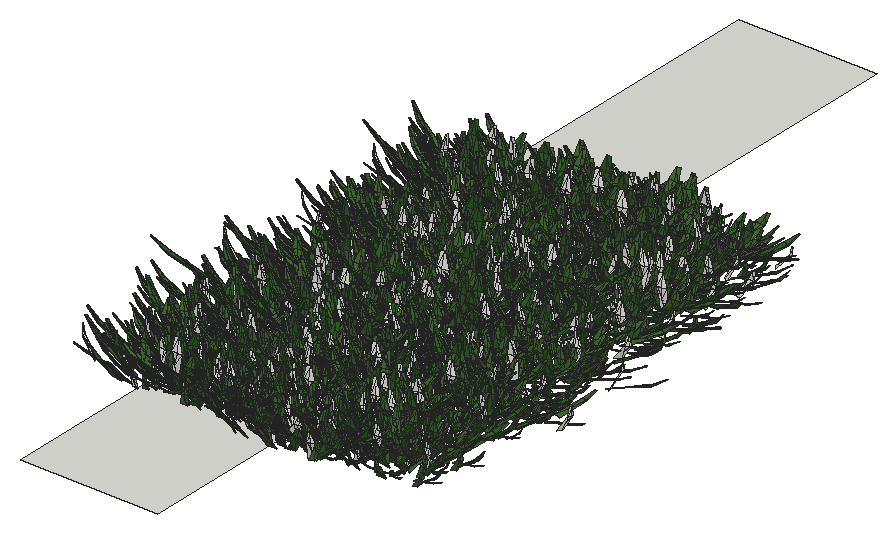
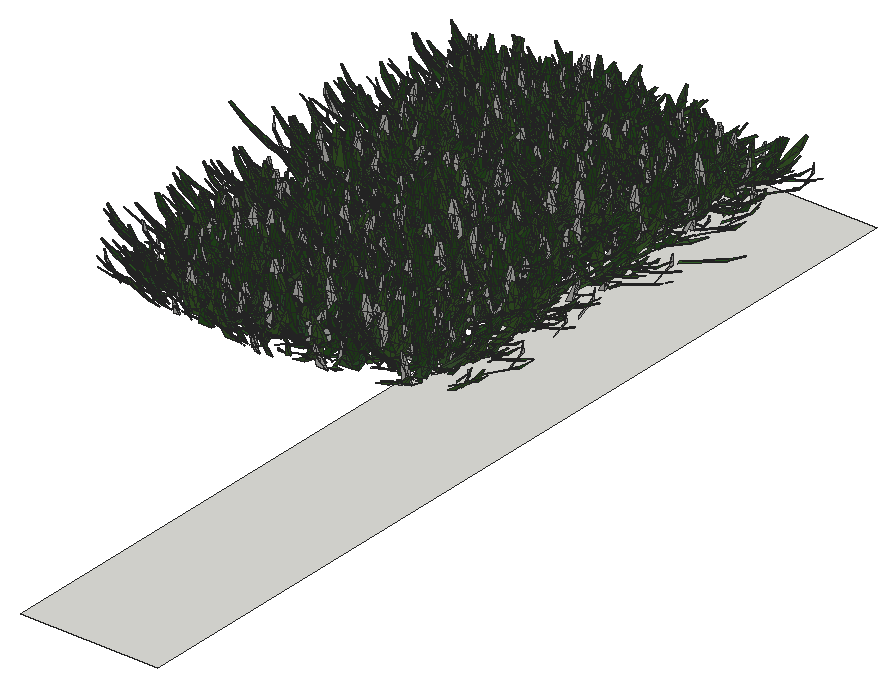
# SketchUp Ruby script. Lengths in inches.
U = 1.inch
M = Sketchup.active_model
def pt(a) = Geom::Point3d.new(a.map { |v| v * U })
def face(e, loops, mat)
  f = e.add_face(loops[0].map { |a| pt(a) })
  loops[1..].each { |l| e.add_face(l.map { |a| pt(a) }).erase! }
  f.material = f.back_material = mat if mat
  f
end
# faces: each face lists its corners as indices into pts; further lists are holes
def faces(e, pts, list, mat = nil) = list.each { |f| face(e, (f[0].is_a?(Array) ? f : [f]).map { |l| l.map { |i| pts[i] } }, mat) }
# xy, xz, yz: faces in a plane at the given z, y or x. An outline is a flat list of corners, or four numbers for a rectangle; further outlines are holes
def ring(l) = l.size == 4 ? [[l[0], l[1]], [l[2], l[1]], [l[2], l[3]], [l[0], l[3]]] : l.each_slice(2).to_a
def flat(e, list, mat, &to3) = list.each { |f| face(e, (f[0].is_a?(Array) ? f : [f]).map { |l| ring(l).map { |u, v| to3.(u, v) } }, mat) }
def xy(e, z, list, mat = nil) = flat(e, list, mat) { |x, y| [x, y, z] }
def xz(e, y, list, mat = nil) = flat(e, list, mat) { |x, z| [x, y, z] }
def yz(e, x, list, mat = nil) = flat(e, list, mat) { |y, z| [x, y, z] }
def lines(e, pts, list) = list.each { |a, b| e.add_line(pt(pts[a]), pt(pts[b])) }
# prism: a flat outline (further loops are holes) pulled along v
def prism(e, loops, v, mat = nil)
  f = face(e, loops, mat); d = Geom::Vector3d.new(v.map { |x| x * U })
  f.pushpull(f.normal.samedirection?(d) ? d.length : -d.length)
end
def box(e, o, s, mat = nil) = prism(e, [[o, [o[0] + s[0], o[1], o[2]], [o[0] + s[0], o[1] + s[1], o[2]], [o[0], o[1] + s[1], o[2]]]], [0, 0, s[2]], mat)
def at(x, y, z, deg = 0) = Geom::Transformation.translation(pt([x, y, z])) * Geom::Transformation.rotation(ORIGIN, Z_AXIS, deg.degrees)
def axes(o, x, y, z) = Geom::Transformation.new([*x, 0, *y, 0, *z, 0, *pt(o).to_a, 1])
def part(name) = M.definitions.add(name)
# library, detail: a bought-in or finely detailed component or shape, given as its bounding box
def library(name, o, s) = part(name).tap { |d| box(d.entities, o, s) }
def detail(e, o, s) = box(e.add_group.entities, o, s)
def put(e, d, t, mat = nil) = e.add_instance(d, t).tap { |i| i.material = mat if mat }
def group(e, t, mat = nil) = e.add_group.tap { |g| g.transformation = t; g.material = mat if mat }.entities
root = M.entities
M.materials.add("Material82").color = [68, 110, 58]
M.materials.add("Material83").color = [48, 90, 38]
M.materials.add("Material84").color = [68, 110, 48]
M.materials.add("Material85").color = [48, 90, 48]
M.materials.add("Material86").color = [58, 110, 58]
M.materials.add("Material87").color = [58, 90, 38]
M.materials.add("Material88").color = [68, 100, 58]
M.materials.add("Material89").color = [48, 100, 38]
c1 = part("grass00")
p = [[-0.6875,0.15,0],[-0.56,0.08,5.52],[-0.04,0.03,2.76],[0.48,-0.02,0],[0.35,-0.02,5.52],[-0.1,-0.14,5.52],
  [-0.12,0.65,8.37],[-0.42,0.65,8.37]]
faces(c1.entities,p,[[0,1,2,3],[3,2,4],[1,5,2],[5,4,2],[1,6,5],[4,5,6],[7,6,1]])
c2 = part("Group16\#1")
put(c2.entities,c1,axes([1.44,-0.61,-0.01],[0.05352,0.12609,0],[-0.10704,0.04543,0.07239],[0.06664,-0.02828,0.11628]),"Material85")
put(c2.entities,c1,axes([0.76,-0.15,-0.01],[0.04676,0.24062,0],[-0.23162,0.04501,0.06642],[0.0652,-0.01267,0.23595]),"Material82")
put(c2.entities,c1,axes([0.79,0.01,-0.01],[-0.00606,0.34651,0],[-0.34381,-0.00602,0.0432],[0.04319,0.00076,0.34386]))
put(c2.entities,c1,axes([1,0.23,-0.01],[-0.07192,0.31144,0],[-0.28722,-0.06632,0.1236],[0.12043,0.02781,0.29478]),"Material84")
put(c2.entities,c1,axes([1.66,0.77,-0.01],[-0.13828,0.29651,0],[-0.21551,-0.1005,0.22471],[0.20365,0.09498,0.23779]),"Material89")
put(c2.entities,c1,axes([0.6875,0.52,-0.01],[-0.18126,0.24051,0],[-0.22746,-0.17142,0.09788],[0.07817,0.05891,0.28481]),"Material84")
put(c2.entities,c1,axes([0.68,0.78,-0.01],[-0.215,0.18688,0],[-0.12385,-0.14248,0.21334],[0.13995,0.16101,0.18878]),"Material82")
put(c2.entities,c1,axes([0.56,1,-0.01],[-0.13756,0.07624,0],[-0.06159,-0.11112,0.0927],[0.04494,0.08108,0.12705]),"Material84")
put(c2.entities,c1,axes([0.2,0.64,-0.01],[-0.23729,0.07254,0],[-0.05711,-0.18681,0.153],[0.04473,0.14632,0.19535]),"Material89")
put(c2.entities,c1,axes([0.0625,0.72,-0.01],[-0.28874,0.02525,0],[-0.02179,-0.24916,0.14647],[0.01276,0.14591,0.25012]),"Material82")
put(c2.entities,c1,axes([-0.08,0.62,-0.01],[-0.34089,-0.04187,0],[0.03255,-0.26504,0.216],[-0.02633,0.21439,0.26703]),"Material89")
put(c2.entities,c1,axes([-0.34,0.98,-0.01],[-0.14314,-0.0493,0],[0.04397,-0.12769,0.06843],[-0.02228,0.0647,0.13505]),"Material89")
put(c2.entities,c1,axes([-0.87,1.45,-0.01],[-0.23488,-0.14114,0],[0.13761,-0.22901,0.06087],[-0.03135,0.05217,0.26717]))
put(c2.entities,c1,axes([-0.72,0.77,-0.01],[-0.14208,-0.13251,0],[0.07209,-0.0773,0.16301],[-0.11118,0.11922,0.1057]),"Material89")
put(c2.entities,c1,axes([-0.62,0.43,-0.01],[-0.14845,-0.21203,0],[0.18654,-0.13061,0.12304],[-0.10079,0.07057,0.22772]),"Material82")
put(c2.entities,c1,axes([-0.68,0.29,-0.01],[-0.13639,-0.32136,0],[0.31723,-0.13464,0.05579],[-0.05136,0.0218,0.34462]),"Material83")
put(c2.entities,c1,axes([-0.64,0.125,-0.01],[-0.0458,-0.23569,0],[0.22124,-0.043,0.08276],[-0.08124,0.01579,0.22538]),"Material86")
put(c2.entities,c1,axes([-1.6,-0.03,-0.01],[0.00576,-0.32897,0],[0.27526,0.00482,0.18018],[-0.18015,-0.00315,0.2753]),"Material84")
put(c2.entities,c1,axes([-1.36,-0.31,-0.01],[0.05718,-0.24765,0],[0.18172,0.04196,0.17267],[-0.16825,-0.03885,0.1865]),"Material89")
put(c2.entities,c1,axes([-1.54,-0.72,-0.01],[0.06537,-0.14017,0],[0.13555,0.06321,0.03939],[-0.0357,-0.01665,0.14956]))
put(c2.entities,c1,axes([-1.19,-0.9,-0.01],[0.09597,-0.12735,0],[0.11214,0.08451,0.07557],[-0.06035,-0.04548,0.14042]),"Material88")
put(c2.entities,c1,axes([-0.47,-0.54,-0.01],[0.11588,-0.10072,0],[0.0618,0.0711,0.12124],[-0.07953,-0.0915,0.0942]))
put(c2.entities,c1,axes([-0.47,-0.84,-0.01],[0.11927,-0.0661,0],[0.06603,0.11913,0.00646],[-0.00313,-0.00565,0.13621]),"Material84")
put(c2.entities,c1,axes([-0.38,-1.24,-0.01],[0.28037,-0.08571,0],[0.0618,0.20215,0.20315],[-0.05939,-0.19428,0.21139]),"Material88")
put(c2.entities,c1,axes([-0.06,-0.66,-0.01],[0.22719,-0.01987,0],[0.01247,0.14255,0.17758],[-0.01547,-0.17691,0.1431]),"Material87")
put(c2.entities,c1,axes([0.11,-0.89,-0.01],[0.14882,0.01828,0],[-0.01058,0.08611,0.12229],[0.01491,-0.12138,0.08676]),"Material85")
put(c2.entities,c1,axes([0.25,-0.72,-0.01],[0.20481,0.07053,0],[-0.06206,0.18022,0.10291],[0.03351,-0.0973,0.1906]),"Material85")
put(c2.entities,c1,axes([0.85,-1.42,-0.01],[0.16481,0.09904,0],[-0.09472,0.15762,0.05616],[0.02893,-0.04814,0.18389]),"Material84")
put(c2.entities,c1,axes([1.01,-1.09,-0.01],[0.21858,0.20385,0],[-0.17495,0.1876,0.15339],[0.10462,-0.11218,0.25652]),"Material89")
put(c2.entities,c1,axes([1.01,-0.71,-0.01],[0.08733,0.12473,0],[-0.06445,0.04512,0.13037],[0.1068,-0.07477,0.07867]),"Material85")
c3 = part("Group15\#1")
put(c3.entities,c2,at(0,0,0))
c4 = part("3darcstudiotree_grass00\#1")
put(c4.entities,c3,at(0,0,0))
xy(root,-42.1875,[[609.09,273.41,626.68,387.84]])
put(root,c4,axes([618.03,286.12,-34.17],[1.73893,-1.7168,0],[3.5493,0.55914,-0.05078],[0.28442,0.04481,1.72798]))
put(root,c4,axes([617.23,283.25,-34.17],[1.27117,1.29221,0],[-3.51403,0.53763,-0.02781],[-0.14445,0.0221,1.57422]))
put(root,c4,axes([618.71,309.98,-34.17],[1.49045,-1.29572,0],[4.01852,0.71892,-0.00454],[0.01627,0.00291,1.30224]))
put(root,c4,axes([617.49,293.86,-34.17],[3.40006,0.04588,0],[-0.15479,1.78412,-0.02332],[-0.00425,0.049,1.80921]))
put(root,c4,axes([617.25,329.67,-34.17],[1.48796,1.33204,0],[-3.50735,0.60935,-0.02705],[-0.13278,0.02307,1.54111]))
put(root,c4,axes([618.95,332.66,-34.17],[-3.4737,0.48099,0],[-1.22806,-1.37939,-0.01418],[-0.03068,-0.03446,1.8149]))
put(root,c4,axes([617.72,322.07,-34.17],[1.0762,1.29593,0],[-3.71861,0.48029,-0.00037],[-0.00166,0.00021,1.37352]))
put(root,c4,axes([619.43,303,-34.17],[-4.57816,0.34958,0],[-0.88534,-1.8033,-0.01839],[-0.0151,-0.03075,1.50803]))
put(root,c4,axes([619.66,291.15,-34.17],[-1.62742,-1.17488,0],[3.69115,-0.79521,-0.05959],[0.21649,-0.04664,1.30502]))
put(root,c4,axes([618.88,320.27,-34.17],[1.77469,-1.16148,0],[2.86416,0.68064,-0.04784],[0.28474,0.06767,1.7418]))
put(root,c4,axes([619.79,326.4375,-34.17],[-0.38907,-1.30448,0],[3.64191,-0.16894,-0.01277],[0.06378,-0.00296,1.38207]))
put(root,c4,axes([618.34,318.48,-34.17],[0.22262,1.70783,0],[-4.21483,0.08545,-0.0387],[-0.20922,0.00424,1.71236]))
put(root,c4,axes([618.17,306.94,-34.17],[1.40686,1.47706,0],[-4.38712,0.6499,-0.05425],[-0.24934,0.03694,1.72469]))
put(root,c4,axes([618.59,335.93,-34.17],[3.74197,-0.40965,0],[1.02528,1.45661,-0.05393],[0.09104,0.12934,1.81331]))
put(root,c4,axes([619.11,289.47,-34.17],[-1.63246,1.63511,0],[-3.4831,-0.54085,-0.00571],[-0.03452,-0.00536,1.8245]))
put(root,c4,axes([619.32,298.92,-34.17],[-0.95146,1.7451,0],[-3.70497,-0.31417,-0.03186],[-0.21482,-0.01822,1.95913]))
put(root,c4,axes([620.37,331.43,-34.17],[3.26505,-0.4107,0],[1.3901,1.71877,-0.05774],[0.0978,0.12093,1.91123]))
put(root,c4,axes([620.2,314.42,-34.17],[2.80643,0.90661,0],[-2.10951,1.0156,-0.00694],[-0.02809,0.01352,1.5947]))
put(root,c4,axes([620.43,296.95,-34.17],[4.57178,0.1006,0],[-0.19659,1.38952,-0.03032],[-0.00983,0.06951,1.54015]))
put(root,c4,axes([622.11,331.34,-34.17],[-3.18088,-0.40858,0],[1.35408,-1.63957,-0.00123],[0.00227,-0.00275,1.95221]))
put(root,c4,axes([622.9375,296.25,-34.17],[-2.17426,-1.31341,0],[3.93463,-1.01304,-0.04707],[0.15585,-0.04013,1.39282]))
put(root,c4,axes([622.58,287.45,-34.17],[-3.35474,0.10257,0],[-0.29043,-1.4774,-0.03359],[-0.01806,-0.09187,1.95875]))
put(root,c4,axes([622.22,318.16,-34.17],[3.26089,-0.9276,0],[2.41726,1.32164,-0.00659],[0.02436,0.01332,1.95827]))
put(root,c4,axes([622.02,283.82,-34.17],[3.92346,-0.38379,0],[1.02863,1.63546,-0.04456],[0.04806,0.07641,1.43455]))
put(root,c4,axes([623.68,313.41,-34.17],[-3.24318,-0.61658,0],[1.47082,-1.20323,-0.00927],[0.0316,-0.02585,1.99366]))
put(root,c4,axes([624.23,293.77,-34.17],[-0.91872,-1.28532,0],[4.49567,-0.49978,-0.01485],[0.07367,-0.00819,1.80381]))
put(root,c4,axes([623.52,307.1,-34.17],[0.6017,-1.37989,0],[3.88457,0.26344,-0.05034],[0.29768,0.02019,1.77282]))
put(root,c4,axes([622.875,285.4,-34.17],[3.93415,-0.89756,0],[1.9948,1.35987,-0.042],[0.11006,0.07503,1.56273]))
put(root,c4,axes([623.05,335.04,-34.17],[-1.11116,1.30676,0],[-3.31516,-0.43843,-0.03292],[-0.23061,-0.0305,1.93659]))
put(root,c4,axes([624.4,319.98,-34.17],[-1.52685,-1.32373,0],[3.20025,-0.57411,-0.03768],[0.23061,-0.04137,1.77164]))
put(root,c4,axes([623.49,325.38,-34.17],[-1.03634,1.43503,0],[-4.07668,-0.45789,-0.05457],[-0.22787,-0.02559,1.37935]))
put(root,c4,axes([624.74,326.875,-34.17],[-3.57412,-0.0033,0],[0.00935,-1.57631,-0.04252],[0.00057,-0.09613,1.71753]))
put(root,c4,axes([624.45,323.15,-34.17],[1.46562,-1.72266,0],[4.03529,0.53396,-0.04434],[0.25483,0.03372,1.93394]))
put(root,c4,axes([623.28,304.17,-34.17],[3.29517,0.70525,0],[-2.24642,1.63243,-0.00178],[-0.00323,0.00235,1.34491]))
put(root,c4,axes([625.18,291.3,-34.17],[-3.95181,0.01249,0],[-0.03447,-1.69649,-0.00779],[-0.00033,-0.01629,1.71052]))
put(root,c4,axes([623.75,332.5625,-34.17],[0.85595,1.34318,0],[-4.39323,0.43542,-0.04255],[-0.19043,0.01887,1.5668]))
put(root,c4,axes([624.81,298.65,-34.17],[2.65299,-0.97546,0],[3.20943,1.35758,-0.02398],[0.06395,0.02705,1.37951]))
put(root,c4,axes([623.97,315.24,-34.17],[-0.08871,1.46443,0],[-4.0853,-0.03849,-0.0357],[-0.16722,-0.00158,1.43525]))
put(root,c4,axes([624.625,302.09,-34.17],[-1.54224,1.54277,0],[-3.96225,-0.61604,-0.03242],[-0.18554,-0.02885,1.96368]))
put(root,c4,axes([625.48,289.625,-34.17],[1.45525,-1.36358,0],[3.3603,0.55776,-0.00467],[0.02235,0.00371,1.41828]))
put(root,c4,axes([624.95,328.28,-34.17],[3.00061,-1.20381,0],[2.59687,1.00673,-0.02297],[0.10061,0.039,1.67632]))
put(root,c4,axes([624.89,338.31,-34.17],[3.81318,-1.10593,0],[2.582,1.38461,-0.02397],[0.05758,0.03088,1.32443]))
put(root,c4,axes([625.95,300.13,-34.17],[-4.06047,-0.30244,0],[0.85134,-1.77769,-0.03943],[0.03436,-0.07175,1.61444]))
put(root,c4,axes([624.44,311.82,-34.17],[4.70379,-0.18713,0],[0.44198,1.72795,-0.01121],[0.00446,0.01743,1.30781]))
put(root,c4,axes([625.31,309.8,-34.17],[4.53982,0.21063,0],[-0.49544,1.66085,-0.02625],[-0.01899,0.06364,1.96735]))
put(root,c4,axes([627.48,287.28,-34.17],[-3.49662,-0.83415,0],[2.45665,-1.60161,-0.00291],[0.00652,-0.00425,1.54121]))
put(root,c4,axes([627.65,296.14,-34.17],[0.98995,-1.43102,0],[4.03348,0.43397,-0.01691],[0.08344,0.00898,1.6028]))
put(root,c4,axes([627.73,319.87,-34.17],[2.00913,-1.08398,0],[3.65765,1.05439,-0.0361],[0.15471,0.0446,1.80295]))
put(root,c4,axes([627.58,333.45,-34.17],[-2.26736,0.9467,0],[-3.26135,-1.21483,-0.01576],[-0.0639,-0.0238,1.87507]))
put(root,c4,axes([627.99,310.1,-34.17],[3.78243,-0.20016,0],[0.50434,1.48226,-0.04419],[0.03105,0.09126,1.50171]))
put(root,c4,axes([629.04,330.47,-34.17],[-3.45253,0.27622,0],[-0.72182,-1.40321,-0.01756],[-0.02267,-0.04407,1.76676]))
put(root,c4,axes([627.88,283.46,-34.17],[3.16343,0.45899,0],[-1.51538,1.62437,-0.05896],[-0.12026,0.12891,1.94308]))
put(root,c4,axes([629.05,335.34,-34.17],[0.78455,-1.57227,0],[3.87046,0.30038,-0.05061],[0.32766,0.02543,1.95081]))
put(root,c4,axes([629.59,314.09,-34.17],[-4.25587,0.04591,0],[-0.1089,-1.57017,-0.04984],[-0.00682,-0.0984,1.49526]))
put(root,c4,axes([629.57,315.32,-34.17],[0.66389,-1.49509,0],[4.57403,0.31589,-0.04237],[0.23153,0.01599,1.93074]))
put(root,c4,axes([629.01,307.87,-34.17],[-2.17136,1.02025,0],[-2.89421,-0.95801,-0.02769],[-0.1122,-0.03714,1.49833]))
put(root,c4,axes([629.1,300.01,-34.17],[-1.21684,1.60263,0],[-3.24686,-0.38342,-0.04102],[-0.25836,-0.03051,1.67021]))
put(root,c4,axes([629.65,298.69,-34.17],[-3.24632,0.41503,0],[-1.13877,-1.38534,-0.02033],[-0.04358,-0.05301,1.92362]))
put(root,c4,axes([628.75,326.37,-34.17],[3.77678,0.27869,0],[-0.6902,1.45473,-0.00485],[-0.00557,0.01174,1.75633]))
put(root,c4,axes([628.62,289.48,-34.17],[0.70399,1.48206,0],[-4.34932,0.32132,-0.00799],[-0.0357,0.00264,1.50733]))
put(root,c4,axes([629.35,303.2,-34.17],[4.36912,-0.54802,0],[1.07763,1.33621,-0.00335],[0.00554,0.00687,1.45436]))
put(root,c4,axes([630.24,337.63,-34.17],[1.61856,-1.20753,0],[3.98562,0.83088,-0.05061],[0.25894,0.05398,1.95538]))
put(root,c4,axes([631.02,284.88,-34.17],[-4.39724,-0.41789,0],[0.97106,-1.58919,-0.03666],[0.03598,-0.05889,1.30149]))
put(root,c4,axes([631.32,291.59,-34.17],[-3.07103,-1.30718,0],[3.25603,-1.18973,-0.02123],[0.06738,-0.02462,1.43939]))
put(root,c4,axes([629.86,318.12,-34.17],[3.97153,-0.13343,0],[0.30373,1.40602,-0.01096],[0.00672,0.03109,1.93666]))
put(root,c4,axes([631.36,340.02,-34.17],[-2.26232,-1.46372,0],[3.35674,-0.80691,-0.05337],[0.23381,-0.0562,1.5119]))
put(root,c4,axes([631.15,324.36,-34.17],[0.94741,-1.42267,0],[3.73003,0.38633,-0.03356],[0.18091,0.01874,1.61101]))
put(root,c4,axes([630.14,294.03,-34.17],[3.9873,-0.15062,0],[0.35569,1.46445,-0.02913],[0.01977,0.08141,1.9903]))
put(root,c4,axes([631.5,311.43,-34.17],[0.11291,-1.83708,0],[4.52912,0.0433,-0.04883],[0.22915,0.00219,1.59403]))
put(root,c4,axes([629.84,304.79,-34.17],[1.39223,1.25256,0],[-3.795,0.65605,-0.01361],[-0.06427,0.01111,1.60179]))
put(root,c4,axes([630.62,322.18,-34.17],[4.35154,-0.63119,0],[1.42423,1.52711,-0.01984],[0.04228,0.04533,1.90869]))
put(root,c4,axes([631.02,328.61,-34.17],[2.81234,1.34734,0],[-2.81254,0.91306,-0.01155],[-0.05543,0.018,1.69697]))
put(root,c4,axes([633.22,301.41,-34.17],[-3.18803,-0.40221,0],[1.38309,-1.70502,-0.00535],[0.00805,-0.00992,1.67969]))
put(root,c4,axes([633.36,309.92,-34.17],[0.12157,-1.62148,0],[4.39568,0.05126,-0.0158],[0.08264,0.00096,1.72451]))
put(root,c4,axes([633.625,289.96,-34.17],[0.05707,-1.33182,0],[4.67038,0.03113,-0.02351],[0.10833,0.00072,1.61343]))
put(root,c4,axes([633.02,297.8125,-34.17],[2.55829,-1.10547,0],[3.21956,1.15881,-0.03913],[0.13719,0.04938,1.55084]))
put(root,c4,axes([633.7,315.66,-34.17],[-4.65824,0.34825,0],[-0.74927,-1.55877,-0.04366],[-0.04609,-0.09588,1.70895]))
put(root,c4,axes([634.02,307.59,-34.17],[-4.52964,-0.09494,0],[0.22898,-1.69903,-0.02618],[0.00745,-0.05528,1.73378]))
put(root,c4,axes([634.36,326.74,-34.17],[-3.60203,-0.72226,0],[1.64221,-1.27378,-0.05096],[0.13667,-0.10601,1.60728]))
put(root,c4,axes([633.12,325.2,-34.17],[3.44825,-0.26897,0],[0.66516,1.32629,-0.00259],[0.00332,0.00662,1.70099]))
put(root,c4,axes([633.45,320.69,-34.17],[3.35413,-0.63199,0],[1.61191,1.33051,-0.01719],[0.04506,0.03719,1.70421]))
put(root,c4,axes([634.74,331.67,-34.17],[-3.59651,-0.44623,0],[1.25179,-1.56915,-0.00258],[0.00335,-0.0042,1.35273]))
put(root,c4,axes([635.05,291.83,-34.17],[-3.14814,-1.33954,0],[3.08708,-1.12839,-0.01903],[0.08494,-0.03105,1.91973]))
put(root,c4,axes([634.04,302.16,-34.17],[-2.16052,1.42464,0],[-3.02099,-0.71254,-0.01081],[-0.04852,-0.01144,1.38013]))
put(root,c4,axes([634.51,335.55,-34.17],[1.98347,-1.087,0],[3.74124,1.06175,-0.05142],[0.23843,0.06767,1.97373]))
put(root,c4,axes([633.61,305.125,-34.17],[1.97793,1.10174,0],[-3.47293,0.96971,-0.06047],[-0.20758,0.05796,1.34144]))
put(root,c4,axes([635.35,329.35,-34.17],[-1.19412,-1.34448,0],[3.1862,-0.44013,-0.02961],[0.14836,-0.02049,1.34337]))
put(root,c4,axes([634.47,296.48,-34.17],[-1.72626,1.58438,0],[-3.31687,-0.56206,-0.02574],[-0.1159,-0.01964,1.32606]))
put(root,c4,axes([634.47,314.18,-34.17],[2.97087,-0.63768,0],[1.76888,1.28171,-0.04084],[0.13668,0.09904,1.94165]))
put(root,c4,axes([636.1,318.24,-34.17],[-2.73035,-0.81396,0],[2.55013,-1.33042,-0.03674],[0.11326,-0.05909,1.62045]))
put(root,c4,axes([636.09,286.92,-34.17],[-4.52935,0.02332,0],[-0.05756,-1.73901,-0.02897],[-0.00164,-0.04958,1.4344]))
put(root,c4,axes([634.95,332.6875,-34.17],[3.47707,-0.28838,0],[0.88445,1.65855,-0.04208],[0.03591,0.06734,1.3356]))
put(root,c4,axes([634.86,283.95,-34.17],[3.17869,1.06939,0],[-2.97014,1.37309,-0.05603],[-0.1904,0.08802,1.79617]))
put(root,c4,axes([636.22,294.24,-34.17],[-2.94959,0.77761,0],[-1.85667,-1.09533,-0.00767],[-0.02785,-0.01643,1.63569]))
put(root,c4,axes([636.52,323.12,-34.17],[1.55533,-1.52655,0],[4.26431,0.67573,-0.03894],[0.20513,0.0325,1.95573]))
put(root,c4,axes([636.37,312.12,-34.17],[2.20471,-1.56419,0],[3.09714,0.67895,-0.02727],[0.12975,0.02844,1.44583]))
put(root,c4,axes([636.79,339.89,-34.17],[0.44293,-1.56057,0],[3.90028,0.17217,-0.04376],[0.2246,0.00991,1.51939]))
put(root,c4,axes([635.82,285.08,-34.17],[4.17705,-0.03481,0],[0.09875,1.84286,-0.00824],[0.00079,0.01483,1.59977]))
put(root,c4,axes([636.39,337.99,-34.17],[-2.26608,1.33318,0],[-3.11704,-0.82402,-0.02214],[-0.10686,-0.02825,1.63462]))
put(root,c4,axes([636.23,281.59,-34.17],[3.74746,0.48768,0],[-1.05117,1.25627,-0.0401],[-0.08448,0.10096,1.69032]))
put(root,c4,axes([638.61,318.45,-34.17],[-4.55367,0.27818,0],[-0.67765,-1.72528,-0.03016],[-0.02264,-0.05764,1.62739]))
put(root,c4,axes([639.5625,305.5625,-34.17],[-1.63823,-1.36099,0],[3.49292,-0.65391,-0.00409],[0.01763,-0.0033,1.3842]))
put(root,c4,axes([639,282.83,-34.17],[-3.4101,0.33219,0],[-0.86784,-1.38556,-0.03348],[-0.045,-0.07185,1.52035]))
put(root,c4,axes([639.43,306.59,-34.17],[2.36777,-1.25491,0],[3.70344,1.08678,-0.00846],[0.02737,0.00803,1.39582]))
put(root,c4,axes([640.24,330.67,-34.17],[-4.42879,-0.33071,0],[0.76141,-1.58586,-0.02653],[0.02727,-0.05679,1.69452]))
put(root,c4,axes([640.23,299,-34.17],[-3.60435,-0.22712,0],[0.60496,-1.49319,-0.01241],[0.00897,-0.02215,1.31731]))
put(root,c4,axes([639.13,311.36,-34.17],[3.96894,-0.58875,0],[1.33194,1.3965,-0.01237],[0.02838,0.02976,1.84855]))
put(root,c4,axes([640.63,286.82,-34.17],[-3.95806,-0.26007,0],[0.56997,-1.34913,-0.01531],[0.01744,-0.04128,1.80136]))
put(root,c4,axes([640.48,291.09,-34.17],[0.93986,-1.61608,0],[3.43783,0.31095,-0.013],[0.09422,0.00852,1.96601]))
put(root,c4,axes([640.89,294.27,-34.17],[-0.9687,-1.6973,0],[3.99206,-0.35436,-0.03143],[0.1527,-0.01355,1.52743]))
put(root,c4,axes([641.2,316.53,-34.17],[-1.5733,-1.53629,0],[3.8056,-0.60614,-0.01424],[0.06159,-0.00981,1.43479]))
put(root,c4,axes([641.05,332.76,-34.17],[-3.45853,-0.30921,0],[0.875,-1.52216,-0.03754],[0.05438,-0.09459,1.94323]))
put(root,c4,axes([640.76,295.6,-34.17],[-0.43954,-1.59759,0],[3.53501,-0.15126,-0.05057],[0.33495,-0.01433,1.77563]))
put(root,c4,axes([639.74,309.33,-34.17],[3.08639,0.66231,0],[-1.76537,1.27948,-0.04213],[-0.09869,0.07153,1.35679]))
put(root,c4,axes([640.95,290.28,-34.17],[2.93587,-1.18133,0],[2.75704,1.06566,-0.0131],[0.05816,0.02248,1.79861]))
put(root,c4,axes([641.8,319.46,-34.17],[-3.47148,-0.32447,0],[1.09042,-1.81447,-0.00987],[0.00954,-0.01587,1.48448]))
put(root,c4,axes([639.98,302.78,-34.17],[3.59479,1.11581,0],[-2.65109,1.32837,-0.01986],[-0.0739,0.03703,1.93312]))
put(root,c4,axes([640.8,285.5625,-34.17],[-0.72391,1.71321,0],[-3.27988,-0.21555,-0.00349],[-0.01869,-0.00123,1.35435]))
put(root,c4,axes([640.8125,337.3125,-34.17],[3.93037,0.00712,0],[-0.01552,1.3324,-0.03904],[-0.00131,0.11261,1.85207]))
put(root,c4,axes([641.82,299.85,-34.17],[1.97331,-1.7001,0],[3.41411,0.61633,-0.04178],[0.21918,0.03957,1.62381]))
put(root,c4,axes([640.96,313.02,-34.17],[3.30561,0.92504,0],[-2.54174,1.41264,-0.05586],[-0.15004,0.08339,1.52805]))
put(root,c4,axes([641.9,329.125,-34.17],[3.0975,-0.44176,0],[1.39811,1.52468,-0.04794],[0.07202,0.07854,1.36124]))
put(root,c4,axes([642.64,327.59,-34.17],[2.99585,-0.78884,0],[2.43675,1.4393,-0.03164],[0.10153,0.05997,1.90074]))
put(root,c4,axes([642.28,335.03,-34.17],[4.2542,-0.55295,0],[1.2277,1.46904,-0.0158],[0.03318,0.0397,1.97161]))
put(root,c4,axes([641.93,325.14,-34.17],[1.7248,1.72946,0],[-3.94677,0.61218,-0.01805],[-0.10059,0.0156,1.90362]))
put(root,c4,axes([641.93,339.14,-34.17],[0.74688,1.42324,0],[-4.33801,0.35406,-0.00233],[-0.01216,0.00099,1.77271]))
put(root,c4,axes([642.48,321.9375,-34.17],[4.44722,-0.53115,0],[1.26492,1.64719,-0.03542],[0.04521,0.05887,1.44036]))
put(root,c4,axes([644.24,305.17,-34.17],[-2.92804,-0.86099,0],[2.52273,-1.33432,-0.01853],[0.05328,-0.02818,1.52144]))
put(root,c4,axes([644.53,316.7,-34.17],[-3.6982,-1.11774,0],[2.6803,-1.37926,-0.01589],[0.04062,-0.0209,1.38765]))
put(root,c4,axes([644.2,322.29,-34.17],[-4.1478,0.13224,0],[-0.279,-1.36104,-0.02584],[-0.01399,-0.06822,1.74304]))
put(root,c4,axes([644.09,329.11,-34.17],[2.38875,-0.89777,0],[2.38741,0.98797,-0.03437],[0.15253,0.06312,1.66865]))
put(root,c4,axes([644.79,333.22,-34.17],[0.38467,-1.72776,0],[3.7527,0.12994,-0.02351],[0.1369,0.00474,1.65028]))
put(root,c4,axes([645.38,339.19,-34.17],[-0.80049,-1.46058,0],[4.26303,-0.36338,-0.06129],[0.24511,-0.02089,1.3376]))
put(root,c4,axes([644.18,300.5,-34.17],[3.0128,0.96923,0],[-2.26467,1.09486,-0.0073],[-0.03331,0.01611,1.93831]))
put(root,c4,axes([646.16,334.76,-34.17],[-4.20928,0.13814,0],[-0.29813,-1.41294,-0.01346],[-0.00713,-0.03379,1.72106]))
put(root,c4,axes([646.4,287.39,-34.17],[-3.15856,-0.38514,0],[1.26271,-1.61061,-0.02785],[0.04659,-0.05943,1.81462]))
put(root,c4,axes([645.73,292.03,-34.17],[-1.513,1.21159,0],[-3.36011,-0.6526,-0.03193],[-0.17356,-0.03371,1.70102]))
put(root,c4,axes([646.87,298.42,-34.17],[-3.75328,0.12847,0],[-0.28677,-1.30306,-0.03872],[-0.02406,-0.10934,1.78675]))
put(root,c4,axes([645.6,337.64,-34.17],[3.29344,0.56908,0],[-1.86687,1.68036,-0.0492],[-0.08744,0.0787,1.54416]))
put(root,c4,axes([645.92,294.05,-34.17],[3.21716,0.40848,0],[-1.16198,1.42335,-0.048],[-0.09517,0.11657,1.83855]))
put(root,c4,axes([647.32,331.08,-34.17],[0.99609,-1.23763,0],[4.45512,0.55768,-0.04397],[0.17141,0.02146,1.43296]))
put(root,c4,axes([648.08,309.81,-34.17],[-1.04498,-1.27032,0],[4.0983,-0.52433,-0.01227],[0.0665,-0.00851,1.83962]))
put(root,c4,axes([647.64,326.91,-34.17],[1.40396,-1.3283,0],[3.66211,0.60201,-0.02113],[0.09939,0.01634,1.51549]))
put(root,c4,axes([646.19,318.02,-34.17],[1.27309,1.64144,0],[-4.4392,0.53549,-0.03143],[-0.12353,0.0149,1.42994]))
put(root,c4,axes([646.92,310.79,-34.17],[3.7109,-0.91214,0],[2.11846,1.34044,-0.04378],[0.13838,0.08756,1.79394]))
put(root,c4,axes([646.61,313.16,-34.17],[3.34228,0.13265,0],[-0.43082,1.68835,-0.00091],[-0.00041,0.00162,1.45853]))
put(root,c4,axes([646.51,302.97,-34.17],[0.73987,1.59354,0],[-4.44696,0.32112,-0.04305],[-0.22862,0.01651,1.82947]))
put(root,c4,axes([646.66,286.08,-34.17],[3.16975,0.46707,0],[-1.43384,1.51339,-0.02415],[-0.05301,0.05595,1.92547]))
put(root,c4,axes([646.95,306.83,-34.17],[0.58066,1.77085,0],[-3.90665,0.19923,-0.04685],[-0.26361,0.01344,1.67517]))
put(root,c4,axes([648.15,319.93,-34.17],[1.02841,-1.31305,0],[3.38391,0.41221,-0.03395],[0.18437,0.02246,1.50895]))
put(root,c4,axes([647.17,283.7,-34.17],[2.81615,0.69239,0],[-1.81737,1.14964,-0.0044],[-0.01183,0.00748,1.30779]))
put(root,c4,axes([647.18,324.42,-34.17],[3.53019,1.19751,0],[-2.61374,1.19838,-0.04839],[-0.15514,0.07113,1.47711]))
put(root,c4,axes([647.28,289.2,-34.17],[3.28885,0.70173,0],[-2.10741,1.53616,-0.00222],[-0.00511,0.00372,1.6055]))
put(root,c4,axes([647.78,296.4,-34.17],[3.3322,0.38036,0],[-1.11394,1.51777,-0.02015],[-0.03056,0.04163,1.63787]))
put(root,c4,axes([650.26,300.84,-34.17],[-2.43541,-1.16543,0],[2.64027,-0.85812,-0.03867],[0.17422,-0.05662,1.49724]))
